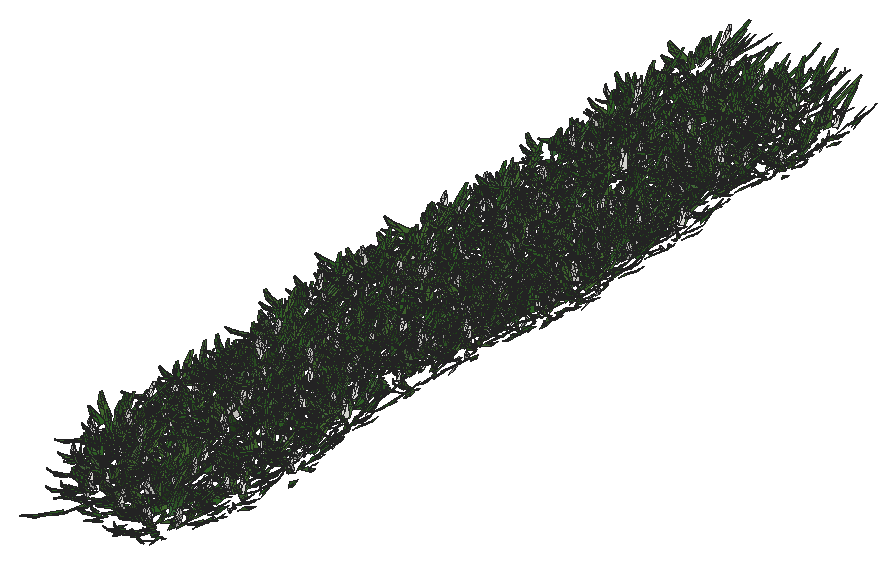
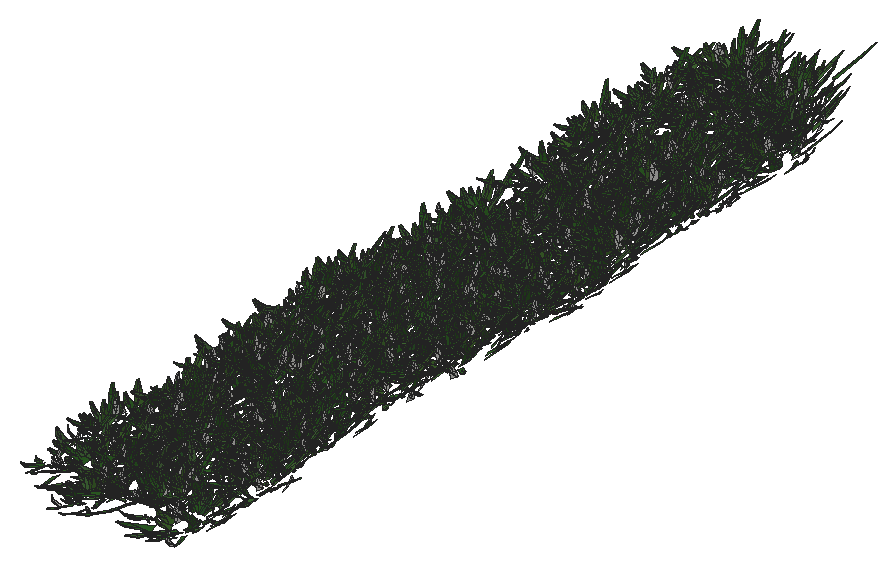
# SketchUp Ruby script. Lengths in inches.
U = 1.inch
M = Sketchup.active_model
def pt(a) = Geom::Point3d.new(a.map { |v| v * U })
def face(e, loops, mat)
  f = e.add_face(loops[0].map { |a| pt(a) })
  loops[1..].each { |l| e.add_face(l.map { |a| pt(a) }).erase! }
  f.material = f.back_material = mat if mat
  f
end
# faces: each face lists its corners as indices into pts; further lists are holes
def faces(e, pts, list, mat = nil) = list.each { |f| face(e, (f[0].is_a?(Array) ? f : [f]).map { |l| l.map { |i| pts[i] } }, mat) }
# xy, xz, yz: faces in a plane at the given z, y or x. An outline is a flat list of corners, or four numbers for a rectangle; further outlines are holes
def ring(l) = l.size == 4 ? [[l[0], l[1]], [l[2], l[1]], [l[2], l[3]], [l[0], l[3]]] : l.each_slice(2).to_a
def flat(e, list, mat, &to3) = list.each { |f| face(e, (f[0].is_a?(Array) ? f : [f]).map { |l| ring(l).map { |u, v| to3.(u, v) } }, mat) }
def xy(e, z, list, mat = nil) = flat(e, list, mat) { |x, y| [x, y, z] }
def xz(e, y, list, mat = nil) = flat(e, list, mat) { |x, z| [x, y, z] }
def yz(e, x, list, mat = nil) = flat(e, list, mat) { |y, z| [x, y, z] }
def lines(e, pts, list) = list.each { |a, b| e.add_line(pt(pts[a]), pt(pts[b])) }
# prism: a flat outline (further loops are holes) pulled along v
def prism(e, loops, v, mat = nil)
  f = face(e, loops, mat); d = Geom::Vector3d.new(v.map { |x| x * U })
  f.pushpull(f.normal.samedirection?(d) ? d.length : -d.length)
end
def box(e, o, s, mat = nil) = prism(e, [[o, [o[0] + s[0], o[1], o[2]], [o[0] + s[0], o[1] + s[1], o[2]], [o[0], o[1] + s[1], o[2]]]], [0, 0, s[2]], mat)
def at(x, y, z, deg = 0) = Geom::Transformation.translation(pt([x, y, z])) * Geom::Transformation.rotation(ORIGIN, Z_AXIS, deg.degrees)
def axes(o, x, y, z) = Geom::Transformation.new([*x, 0, *y, 0, *z, 0, *pt(o).to_a, 1])
def part(name) = M.definitions.add(name)
# library, detail: a bought-in or finely detailed component or shape, given as its bounding box
def library(name, o, s) = part(name).tap { |d| box(d.entities, o, s) }
def detail(e, o, s) = box(e.add_group.entities, o, s)
def put(e, d, t, mat = nil) = e.add_instance(d, t).tap { |i| i.material = mat if mat }
def group(e, t, mat = nil) = e.add_group.tap { |g| g.transformation = t; g.material = mat if mat }.entities
root = M.entities
M.materials.add("Material10").color = [48, 90, 38]
M.materials.add("Material11").color = [68, 110, 48]
M.materials.add("Material12").color = [48, 90, 48]
M.materials.add("Material13").color = [58, 110, 58]
M.materials.add("Material14").color = [58, 90, 38]
M.materials.add("Material15").color = [68, 100, 58]
M.materials.add("Material16").color = [48, 100, 38]
M.materials.add("Material9").color = [68, 110, 58]
c1 = part("grass00")
p = [[-0.6875,0.15,0],[-0.56,0.08,5.52],[-0.04,0.03,2.76],[0.48,-0.02,0],[0.35,-0.02,5.52],[-0.1,-0.14,5.52],
  [-0.12,0.65,8.37],[-0.42,0.65,8.37]]
faces(c1.entities,p,[[0,1,2,3],[3,2,4],[1,5,2],[5,4,2],[1,6,5],[4,5,6],[7,6,1]])
c2 = part("Group16\#1")
put(c2.entities,c1,axes([1.44,-0.61,-0.01],[0.05352,0.12609,0],[-0.10704,0.04543,0.07239],[0.06664,-0.02828,0.11628]),"Material12")
put(c2.entities,c1,axes([0.76,-0.15,-0.01],[0.04676,0.24062,0],[-0.23162,0.04501,0.06642],[0.0652,-0.01267,0.23595]),"Material9")
put(c2.entities,c1,axes([0.79,0.01,-0.01],[-0.00606,0.34651,0],[-0.34381,-0.00602,0.0432],[0.04319,0.00076,0.34386]))
put(c2.entities,c1,axes([1,0.23,-0.01],[-0.07192,0.31144,0],[-0.28722,-0.06632,0.1236],[0.12043,0.02781,0.29478]),"Material11")
put(c2.entities,c1,axes([1.66,0.77,-0.01],[-0.13828,0.29651,0],[-0.21551,-0.1005,0.22471],[0.20365,0.09498,0.23779]),"Material16")
put(c2.entities,c1,axes([0.6875,0.52,-0.01],[-0.18126,0.24051,0],[-0.22746,-0.17142,0.09788],[0.07817,0.05891,0.28481]),"Material11")
put(c2.entities,c1,axes([0.68,0.78,-0.01],[-0.215,0.18688,0],[-0.12385,-0.14248,0.21334],[0.13995,0.16101,0.18878]),"Material9")
put(c2.entities,c1,axes([0.56,1,-0.01],[-0.13756,0.07624,0],[-0.06159,-0.11112,0.0927],[0.04494,0.08108,0.12705]),"Material11")
put(c2.entities,c1,axes([0.2,0.64,-0.01],[-0.23729,0.07254,0],[-0.05711,-0.18681,0.153],[0.04473,0.14632,0.19535]),"Material16")
put(c2.entities,c1,axes([0.0625,0.72,-0.01],[-0.28874,0.02525,0],[-0.02179,-0.24916,0.14647],[0.01276,0.14591,0.25012]),"Material9")
put(c2.entities,c1,axes([-0.08,0.62,-0.01],[-0.34089,-0.04187,0],[0.03255,-0.26504,0.216],[-0.02633,0.21439,0.26703]),"Material16")
put(c2.entities,c1,axes([-0.34,0.98,-0.01],[-0.14314,-0.0493,0],[0.04397,-0.12769,0.06843],[-0.02228,0.0647,0.13505]),"Material16")
put(c2.entities,c1,axes([-0.87,1.45,-0.01],[-0.23488,-0.14114,0],[0.13761,-0.22901,0.06087],[-0.03135,0.05217,0.26717]))
put(c2.entities,c1,axes([-0.72,0.77,-0.01],[-0.14208,-0.13251,0],[0.07209,-0.0773,0.16301],[-0.11118,0.11922,0.1057]),"Material16")
put(c2.entities,c1,axes([-0.62,0.43,-0.01],[-0.14845,-0.21203,0],[0.18654,-0.13061,0.12304],[-0.10079,0.07057,0.22772]),"Material9")
put(c2.entities,c1,axes([-0.68,0.29,-0.01],[-0.13639,-0.32136,0],[0.31723,-0.13464,0.05579],[-0.05136,0.0218,0.34462]),"Material10")
put(c2.entities,c1,axes([-0.64,0.125,-0.01],[-0.0458,-0.23569,0],[0.22124,-0.043,0.08276],[-0.08124,0.01579,0.22538]),"Material13")
put(c2.entities,c1,axes([-1.6,-0.03,-0.01],[0.00576,-0.32897,0],[0.27526,0.00482,0.18018],[-0.18015,-0.00315,0.2753]),"Material11")
put(c2.entities,c1,axes([-1.36,-0.31,-0.01],[0.05718,-0.24765,0],[0.18172,0.04196,0.17267],[-0.16825,-0.03885,0.1865]),"Material16")
put(c2.entities,c1,axes([-1.54,-0.72,-0.01],[0.06537,-0.14017,0],[0.13555,0.06321,0.03939],[-0.0357,-0.01665,0.14956]))
put(c2.entities,c1,axes([-1.19,-0.9,-0.01],[0.09597,-0.12735,0],[0.11214,0.08451,0.07557],[-0.06035,-0.04548,0.14042]),"Material15")
put(c2.entities,c1,axes([-0.47,-0.54,-0.01],[0.11588,-0.10072,0],[0.0618,0.0711,0.12124],[-0.07953,-0.0915,0.0942]))
put(c2.entities,c1,axes([-0.47,-0.84,-0.01],[0.11927,-0.0661,0],[0.06603,0.11913,0.00646],[-0.00313,-0.00565,0.13621]),"Material11")
put(c2.entities,c1,axes([-0.38,-1.24,-0.01],[0.28037,-0.08571,0],[0.0618,0.20215,0.20315],[-0.05939,-0.19428,0.21139]),"Material15")
put(c2.entities,c1,axes([-0.06,-0.66,-0.01],[0.22719,-0.01987,0],[0.01247,0.14255,0.17758],[-0.01547,-0.17691,0.1431]),"Material14")
put(c2.entities,c1,axes([0.11,-0.89,-0.01],[0.14882,0.01828,0],[-0.01058,0.08611,0.12229],[0.01491,-0.12138,0.08676]),"Material12")
put(c2.entities,c1,axes([0.25,-0.72,-0.01],[0.20481,0.07053,0],[-0.06206,0.18022,0.10291],[0.03351,-0.0973,0.1906]),"Material12")
put(c2.entities,c1,axes([0.85,-1.42,-0.01],[0.16481,0.09904,0],[-0.09472,0.15762,0.05616],[0.02893,-0.04814,0.18389]),"Material11")
put(c2.entities,c1,axes([1.01,-1.09,-0.01],[0.21858,0.20385,0],[-0.17495,0.1876,0.15339],[0.10462,-0.11218,0.25652]),"Material16")
put(c2.entities,c1,axes([1.01,-0.71,-0.01],[0.08733,0.12473,0],[-0.06445,0.04512,0.13037],[0.1068,-0.07477,0.07867]),"Material12")
c3 = part("Group15\#1")
put(c3.entities,c2,at(0,0,0))
c4 = part("3darcstudiotree_grass00\#1")
put(c4.entities,c3,at(0,0,0))
put(root,c4,axes([846.08,365.22,12.99],[1.06369,-5.76804,0],[2.34649,2.26106,-0.03331],[0.13333,0.12847,1.51731]))
put(root,c4,axes([846.18,479.74,12.99],[0.45259,5.87694,0],[-3.26833,1.31518,-0.06022],[-0.23227,0.09347,1.78296]))
put(root,c4,axes([846.2,370.94,12.99],[1.45402,4.55379,0],[-2.35041,3.92143,-0.05552],[-0.15671,0.26146,1.39481]))
put(root,c4,axes([847.63,497.58,12.99],[-1.00824,-6.55152,0],[2.51742,-2.02434,-0.03242],[0.11179,-0.0899,1.33794]))
put(root,c4,axes([848.5,380.8125,12.99],[-3.32323,0.92593,0],[-0.32804,-6.15195,-0.03065],[-0.01972,-0.36975,1.97713]))
put(root,c4,axes([848.83,465.13,12.99],[-2.33029,-1.96474,0],[1.16034,-7.19112,-0.02933],[0.03799,-0.23541,1.72129]))
put(root,c4,axes([847.89,502.63,12.99],[3.21155,0.85953,0],[-0.39145,7.64247,-0.02723],[-0.01102,0.21518,1.60719]))
put(root,c4,axes([848.18,289.78,12.99],[2.86445,-0.82084,0],[0.41094,7.49322,-0.03701],[0.02027,0.36959,1.99511]))
put(root,c4,axes([848,405.99,12.99],[2.95868,3.40563,0],[-1.44175,6.54478,-0.03278],[-0.06316,0.28671,1.8841]))
put(root,c4,axes([848.98,375.9,12.99],[1.21855,-5.78751,0],[3.1286,3.44196,-0.06017],[0.19802,0.21785,1.73941]))
put(root,c4,axes([848.31,448.79,12.99],[2.69698,1.04179,0],[-0.45125,6.10404,-0.04218],[-0.0351,0.4748,1.85529]))
put(root,c4,axes([849.4,316.99,12.99],[-0.81503,-5.65935,0],[3.10311,-2.33512,-0.05688],[0.2199,-0.16548,1.82396]))
put(root,c4,axes([848.26,357.72,12.99],[3.10556,1.6743,0],[-0.67424,6.53475,-0.02883],[-0.03024,0.29312,1.84132]))
put(root,c4,axes([848.99,310.21,12.99],[2.13184,-3.94964,0],[2.03475,5.73869,-0.02341],[0.0529,0.14921,1.59067]))
put(root,c4,axes([849.87,327.62,12.99],[-2.25962,-3.55393,0],[1.58703,-5.27249,-0.02104],[0.05386,-0.17895,1.73448]))
put(root,c4,axes([849.875,457.09,12.99],[-1.95242,-3.89116,0],[1.88937,-4.95355,-0.03875],[0.11017,-0.28885,1.70607]))
put(root,c4,axes([849.33,346.31,12.99],[1.84633,-3.73447,0],[2.12858,5.4989,-0.04815],[0.14229,0.36759,1.9649]))
put(root,c4,axes([849.15,475.27,12.99],[2.63938,2.75355,0],[-1.03955,5.20668,-0.03533],[-0.07966,0.39899,1.86502]))
put(root,c4,axes([849.78,394.45,12.99],[2.77698,1.25039,0],[-0.63996,7.42652,-0.03192],[-0.01976,0.22931,1.45488]))
put(root,c4,axes([850.04,428.51,12.99],[-0.33187,6.17881,0],[-2.97957,-0.83623,-0.03564],[-0.14689,-0.04123,1.71014]))
put(root,c4,axes([849.88,423.01,12.99],[1.88972,4.62995,0],[-2.56011,5.45989,-0.03325],[-0.08097,0.17268,1.59934]))
put(root,c4,axes([851.5,405.58,12.99],[0.21539,-7.71794,0],[2.95559,0.431,-0.05413],[0.18491,0.02696,1.39055]))
put(root,c4,axes([851.65,343.35,12.99],[0.44599,-7.88278,0],[3.43149,1.01446,-0.05291],[0.14746,0.0436,1.33374]))
put(root,c4,axes([851.93,393.51,12.99],[1.99767,-5.75199,0],[2.71363,4.92449,-0.06314],[0.13539,0.2457,1.30132]))
put(root,c4,axes([852,321.69,12.99],[0.51895,6.13984,0],[-2.64873,1.16979,-0.03785],[-0.14312,0.06321,1.42505]))
put(root,c4,axes([853.47,336.67,12.99],[-2.97565,-3.89676,0],[1.54592,-6.16836,-0.04075],[0.07384,-0.29465,1.55523]))
put(root,c4,axes([853.5,456.88,12.99],[-0.62688,-5.64888,0],[2.8559,-1.65605,-0.05601],[0.24214,-0.14041,1.80254]))
put(root,c4,axes([853.51,386.74,12.99],[1.87221,-4.7946,0],[2.54876,5.20039,-0.02458],[0.06994,0.14271,1.78746]))
put(root,c4,axes([854.24,441.14,12.99],[-2.80442,-2.07275,0],[1.02319,-7.23363,-0.04655],[0.0496,-0.35067,1.58019]))
put(root,c4,axes([853.31,288.82,12.99],[2.65285,-1.87873,0],[0.74671,5.50944,-0.04073],[0.05006,0.36938,1.43775]))
put(root,c4,axes([853.33,281.66,12.99],[1.13363,5.60093,0],[-3.05552,3.23148,-0.03574],[-0.13437,0.1421,1.91331]))
put(root,c4,axes([853.67,468.9,12.99],[3.14674,3.47141,0],[-1.27001,6.01543,-0.05424],[-0.08028,0.38023,1.36476]))
put(root,c4,axes([854.51,371.89,12.99],[0.93873,-6.42371,0],[2.31185,1.76531,-0.03453],[0.17252,0.13174,1.76116]))
put(root,c4,axes([854.56,274.28,12.99],[0.65379,5.49988,0],[-2.52465,1.56816,-0.02204],[-0.11086,0.06886,1.87051]))
put(root,c4,axes([855.72,335.64,12.99],[-3.16702,-0.15371,0],[0.065,-6.99788,-0.04949],[0.00478,-0.51432,1.9102]))
put(root,c4,axes([856.45,461.74,12.99],[-1.32807,-5.2436,0],[2.60307,-3.44493,-0.02105],[0.08579,-0.11354,1.94345]))
put(root,c4,axes([856.77,439.38,12.99],[-1.64718,-5.90379,0],[2.56899,-3.74523,-0.04256],[0.13378,-0.19503,1.55835]))
put(root,c4,axes([855.86,488.52,12.99],[2.4677,-0.18322,0],[0.11122,7.82696,-0.05593],[0.0062,0.43627,1.60461]))
put(root,c4,axes([857.21,498.3,12.99],[-0.46545,-5.51402,0],[3.35853,-1.48134,-0.02161],[0.08848,-0.03903,1.95654]))
put(root,c4,axes([856.1,422.64,12.99],[0.68004,5.56927,0],[-2.40844,1.53666,-0.02635],[-0.10703,0.06829,1.4463]))
put(root,c4,axes([856.125,412.66,12.99],[2.75541,4.09981,0],[-1.44402,5.07109,-0.02904],[-0.07736,0.27168,1.7729]))
put(root,c4,axes([856.4,348.9375,12.99],[2.26086,2.51617,0],[-1.50969,7.08808,-0.05845],[-0.08327,0.39093,1.53958]))
put(root,c4,axes([857.63,307.67,12.99],[-3.30927,2.34914,0],[-0.81792,-6.02062,-0.03919],[-0.05215,-0.38386,1.69748]))
put(root,c4,axes([856.8,384.55,12.99],[2.97213,-0.50695,0],[0.20315,6.22325,-0.02534],[0.00797,0.24406,1.58232]))
put(root,c4,axes([857.21,283.69,12.99],[2.64295,-1.66108,0],[0.70112,5.82902,-0.03828],[0.04397,0.36554,1.57185]))
put(root,c4,axes([857.09,396.49,12.99],[2.73919,1.69577,0],[-0.71084,5.99975,-0.0432],[-0.04593,0.38771,1.51727]))
put(root,c4,axes([857.64,291.9375,12.99],[-1.59312,5.61237,0],[-2.64617,-3.92486,-0.05659],[-0.15346,-0.22762,1.39892]))
put(root,c4,axes([858.4375,374.95,12.99],[2.07615,-3.40292,0],[1.74164,5.55226,-0.04704],[0.11406,0.36363,1.70604]))
put(root,c4,axes([858.44,354.125,12.99],[3.18751,0.943,0],[-0.44534,7.86574,-0.04718],[-0.01874,0.3309,1.4726]))
put(root,c4,axes([858.63,299.875,12.99],[0.62532,7.4975,0],[-2.55479,1.11339,-0.03349],[-0.14821,0.06459,1.60736]))
put(root,c4,axes([858.61,328.54,12.99],[2.78691,3.36476,0],[-1.29729,5.61451,-0.05015],[-0.11211,0.48519,1.82381]))
put(root,c4,axes([859.75,387.16,12.99],[2.35938,-4.85445,0],[1.80036,4.57218,-0.02235],[0.07834,0.19896,1.93391]))
put(root,c4,axes([860.79,269.33,12.99],[1.03895,-7.06461,0],[3.15067,2.42111,-0.02131],[0.07526,0.05783,1.69918]))
put(root,c4,axes([860.32,329.62,12.99],[1.78329,-6.04262,0],[2.25042,3.47028,-0.04469],[0.18181,0.28036,1.8275]))
put(root,c4,axes([861.14,403.99,12.99],[-2.1541,-4.78139,0],[1.96653,-4.62931,-0.03796],[0.10802,-0.25428,1.58175]))
put(root,c4,axes([859.98,466.62,12.99],[-0.03905,5.59302,0],[-3.37157,-0.123,-0.04794],[-0.17064,-0.00623,1.64652]))
put(root,c4,axes([860.78,417.76,12.99],[1.18779,-6.50536,0],[2.63647,2.51534,-0.05171],[0.20007,0.19088,1.64301]))
put(root,c4,axes([860.42,484.72,12.99],[0.34647,5.87607,0],[-3.16065,0.97379,-0.05207],[-0.21092,0.06498,1.7882]))
put(root,c4,axes([861.61,306.74,12.99],[-2.22021,-5.6511,0],[2.49209,-5.11599,-0.05274],[0.16966,-0.34829,1.98669]))
put(root,c4,axes([860.97,456.35,12.99],[3,1.63244,0],[-0.75172,7.21848,-0.06215],[-0.05278,0.50679,1.63292]))
put(root,c4,axes([862.3125,429.31,12.99],[-2.4368,-3.09441,0],[1.60655,-6.61061,-0.02959],[0.05226,-0.21506,1.65043]))
put(root,c4,axes([861.14,450.09,12.99],[1.09008,5.94814,0],[-2.83436,2.71417,-0.03717],[-0.13159,0.12601,1.61797]))
put(root,c4,axes([861.15,365.25,12.99],[2.15587,4.20517,0],[-1.86376,4.99268,-0.03219],[-0.10025,0.26855,1.88986]))
put(root,c4,axes([862.625,440.88,12.99],[-3.26232,-2.86014,0],[1.20503,-7.18193,-0.02874],[0.02985,-0.17791,1.33872]))
put(root,c4,axes([862.22,338.99,12.99],[3.03096,-2.26489,0],[0.92784,6.488,-0.04269],[0.06267,0.43825,1.93529]))
put(root,c4,axes([862.67,317.89,12.99],[2.03931,-4.55463,0],[2.25979,5.28691,-0.03867],[0.1061,0.24824,1.7417]))
put(root,c4,axes([864.13,401.76,12.99],[-2.91157,-4.36753,0],[1.37492,-4.78932,-0.04657],[0.13679,-0.47648,1.84036]))
put(root,c4,axes([863.91,270.64,12.99],[0.97376,-6.54554,0],[2.91638,2.26702,-0.01889],[0.08323,0.0647,1.96679]))
put(root,c4,axes([863.84,430.42,12.99],[1.88791,-4.76604,0],[2.09608,4.33845,-0.04299],[0.13117,0.27149,1.59659]))
put(root,c4,axes([864.51,264.94,12.99],[-2.24252,-6.03591,0],[2.28388,-4.43375,-0.05304],[0.19219,-0.37311,1.95407]))
put(root,c4,axes([863.99,449.02,12.99],[-1.55822,6.01772,0],[-2.59774,-3.51477,-0.03668],[-0.15095,-0.20424,1.98009]))
put(root,c4,axes([864.28,343.09,12.99],[-2.29812,5.55657,0],[-1.95842,-4.23231,-0.02847],[-0.07859,-0.16983,1.40417]))
put(root,c4,axes([865.0625,385.5625,12.99],[-3.35624,0.65398,0],[-0.22542,-6.04474,-0.04632],[-0.02051,-0.54987,1.89764]))
put(root,c4,axes([865.07,419.13,12.99],[-0.90881,5.87798,0],[-2.31035,-1.86649,-0.03966],[-0.15425,-0.12462,1.38647]))
put(root,c4,axes([865.43,367.76,12.99],[-2.58772,5.27673,0],[-1.86753,-4.78548,-0.04505],[-0.10853,-0.2781,1.39266]))
put(root,c4,axes([866.125,408.51,12.99],[-1.00456,-5.95255,0],[2.82963,-2.49521,-0.03571],[0.15413,-0.13592,1.92492]))
put(root,c4,axes([865.09,496.71,12.99],[1.44814,6.075,0],[-2.47408,3.08166,-0.025],[-0.11319,0.14099,1.99255]))
put(root,c4,axes([866.3125,374.3,12.99],[-3.03706,0.21927,0],[-0.09301,-6.73134,-0.03959],[-0.00511,-0.36973,1.65212]))
put(root,c4,axes([865.2,333.54,12.99],[2.0574,6.068,0],[-2.66536,4.72208,-0.03267],[-0.1083,0.19187,1.93988]))
put(root,c4,axes([865.32,480.65,12.99],[1.0519,6.52766,0],[-3.10051,2.61067,-0.04046],[-0.13074,0.11008,1.56076]))
put(root,c4,axes([865.4,315.18,12.99],[0.01985,5.9818,0],[-3.45212,0.05986,-0.03677],[-0.10753,0.00186,1.38481]))
put(root,c4,axes([866.68,280.02,12.99],[-2.88358,-0.6118,0],[0.31664,-7.79826,-0.06502],[0.01826,-0.44966,1.42798]))
put(root,c4,axes([866.74,308.83,12.99],[1.01643,-7.0272,0],[3.11902,2.35731,-0.04027],[0.1453,0.10982,1.71232]))
put(root,c4,axes([868.36,363.89,12.99],[-0.70141,-5.97923,0],[3.35556,-2.05683,-0.04199],[0.15153,-0.09288,1.7807]))
put(root,c4,axes([868.625,391.23,12.99],[-1.89539,-4.49691,0],[2.16024,-4.75765,-0.03217],[0.08926,-0.19659,1.58546]))
put(root,c4,axes([868.4,308.07,12.99],[-3.1313,1.31472,0],[-0.62999,-7.8402,-0.05609],[-0.04113,-0.51187,1.94158]))
put(root,c4,axes([868.59,349.82,12.99],[-2.83779,-3.28018,0],[1.1007,-4.97574,-0.0255],[0.06682,-0.30206,1.94297]))
put(root,c4,axes([868.34,470.72,12.99],[-2.63853,4.19895,0],[-1.87852,-6.16795,-0.02528],[-0.05662,-0.18591,1.76765]))
put(root,c4,axes([868.16,292.33,12.99],[0.10307,6.4841,0],[-2.60811,0.21663,-0.04285],[-0.21858,0.01816,1.82733]))
put(root,c4,axes([868.29,460.95,12.99],[2.50531,-1.67127,0],[0.93841,7.35041,-0.04654],[0.03812,0.29858,1.34343]))
put(root,c4,axes([868.1,495.49,12.99],[2.68458,2.75681,0],[-1.10476,5.62136,-0.04301],[-0.08005,0.40733,1.6797]))
put(root,c4,axes([868.52,353.45,12.99],[2.60889,-2.1734,0],[1.10499,6.93076,-0.06136],[0.08576,0.53791,1.80687]))
put(root,c4,axes([869.98,284.06,12.99],[-3.1777,2.21789,0],[-0.99385,-7.44046,-0.03433],[-0.02906,-0.21757,1.35329]))
put(root,c4,axes([869.83,408.75,12.99],[-2.2266,5.00695,0],[-1.83096,-4.25454,-0.0233],[-0.08368,-0.19444,1.83382]))
put(root,c4,axes([869.87,327.39,12.99],[-0.4769,5.50254,0],[-3.02986,-1.37211,-0.03573],[-0.13861,-0.06277,1.67549]))
put(root,c4,axes([870.34,372.19,12.99],[-0.6659,7.19493,0],[-3.288,-1.59009,-0.05558],[-0.1877,-0.09077,1.59125]))
put(root,c4,axes([870.86,475.71,12.99],[1.24347,-6.30598,0],[2.24288,2.31096,-0.02223],[0.09784,0.10081,1.62899]))
put(root,c4,axes([872.16,348.43,12.99],[-1.18537,-5.54659,0],[2.44574,-2.73113,-0.0349],[0.1548,-0.17286,1.84302]))
put(root,c4,axes([872.59,405.5,12.99],[-2.8541,-0.0395,0],[0.02062,-7.78505,-0.0591],[0.00117,-0.44044,1.52309]))
put(root,c4,axes([872.74,387.25,12.99],[-3.17891,-0.60485,0],[0.24844,-6.82268,-0.036],[0.01418,-0.38953,1.9513]))
put(root,c4,axes([872.64,506.55,12.99],[0.98174,-5.21568,0],[2.70185,2.65738,-0.02985],[0.10494,0.10321,1.54439]))
put(root,c4,axes([872.42,436.46,12.99],[0.61942,-5.96717,0],[2.37092,1.286,-0.04624],[0.26261,0.14244,1.95114]))
put(root,c4,axes([872.41,478.23,12.99],[-1.50219,6.01734,0],[-2.18613,-2.85168,-0.04437],[-0.16348,-0.21326,1.46464]))
put(root,c4,axes([873.08,264.28,12.99],[0.90473,-6.6234,0],[3.21141,2.29213,-0.04262],[0.16012,0.11428,1.81655]))
put(root,c4,axes([873.125,318.22,12.99],[-1.81586,6.81794,0],[-2.31926,-3.22763,-0.03488],[-0.10964,-0.15258,1.37068]))
put(root,c4,axes([872.79,339.07,12.99],[2.50071,-0.75735,0],[0.34878,6.01755,-0.04905],[0.02621,0.45221,1.48186]))
put(root,c4,axes([873.25,283.78,12.99],[2.37117,-2.04607,0],[0.95251,5.76786,-0.04981],[0.08018,0.48553,1.68613]))
put(root,c4,axes([874.18,395.51,12.99],[-1.52422,-6.19086,0],[2.53637,-3.26297,-0.05229],[0.18805,-0.24192,1.64764]))
put(root,c4,axes([874.25,327.95,12.99],[0.30354,-5.67688,0],[3.18511,0.8899,-0.02785],[0.09403,0.02627,1.49696]))
put(root,c4,axes([873.58,356.19,12.99],[-1.62139,7.1048,0],[-2.97912,-3.55246,-0.04188],[-0.152,-0.18125,1.88687]))
put(root,c4,axes([873.13,450.1,12.99],[2.13282,3.97865,0],[-1.89051,5.29544,-0.03119],[-0.09156,0.25647,1.90467]))
put(root,c4,axes([873.97,496.93,12.99],[-1.35304,6.81193,0],[-2.25958,-2.34517,-0.0444],[-0.19334,-0.20067,1.62807]))
put(root,c4,axes([874.22,418.82,12.99],[-1.67634,5.8436,0],[-2.79431,-4.18852,-0.05216],[-0.12461,-0.18678,1.30947]))
put(root,c4,axes([874.22,427.97,12.99],[-1.36273,6.90676,0],[-3.15633,-3.25402,-0.03185],[-0.11129,-0.11473,1.82087]))
put(root,c4,axes([874.28,309.18,12.99],[1.53536,4.3387,0],[-1.94807,3.60213,-0.02717],[-0.11192,0.20694,1.82093]))
put(root,c4,axes([874.36,271.34,12.99],[2.55774,1.63282,0],[-0.65651,5.37358,-0.03829],[-0.04318,0.35346,1.40372]))
put(root,c4,axes([874.74,469.97,12.99],[2.93849,-1.27374,0],[0.64821,7.81379,-0.05959],[0.03631,0.43776,1.56123]))
put(root,c4,axes([874.83,484.42,12.99],[0.60231,7.5978,0],[-3.28321,1.35999,-0.02342],[-0.08595,0.0356,1.70718]))
put(root,c4,axes([876.38,269.85,12.99],[-2.66911,-1.68953,0],[0.88763,-7.32722,-0.02644],[0.02949,-0.24342,1.9068]))
put(root,c4,axes([876.91,440.8,12.99],[-2.87219,-3.40969,0],[1.49679,-6.58817,-0.03725],[0.05993,-0.26378,1.55507]))
put(root,c4,axes([876.32,495.27,12.99],[-2.0005,6.23176,0],[-2.68773,-4.50835,-0.06171],[-0.18748,-0.31448,1.72322]))
put(root,c4,axes([876.13,465.47,12.99],[1.26204,4.81756,0],[-2.1346,2.92191,-0.04808],[-0.22521,0.30828,1.86326]))
put(root,c4,axes([876.11,391.07,12.99],[3.24405,-0.90953,0],[0.31828,5.93172,-0.03723],[0.01655,0.30849,1.30959]))
put(root,c4,axes([877.49,404.12,12.99],[-1.60999,-5.29002,0],[2.62708,-4.17777,-0.03629],[0.0981,-0.156,1.44541]))
put(root,c4,axes([877.5625,383.13,12.99],[-1.72268,-4.15908,0],[2.53682,-5.49039,-0.06171],[0.15262,-0.3303,1.63202]))
put(root,c4,axes([877.53,431.28,12.99],[-2.01727,3.38084,0],[-1.50139,-4.68098,-0.03589],[-0.1176,-0.36666,1.93035]))
put(root,c4,axes([877.49,414.09,12.99],[-1.11528,6.38022,0],[-2.67266,-2.44117,-0.0529],[-0.19703,-0.17997,1.58349]))
put(root,c4,axes([877.12,334.69,12.99],[1.02935,6.07343,0],[-2.35562,2.08612,-0.02409],[-0.10419,0.09227,1.60735]))
put(root,c4,axes([877.03,281.8125,12.99],[3.38432,1.80751,0],[-0.5848,5.72145,-0.04207],[-0.0361,0.3532,1.32997]))
put(root,c4,axes([877.95,316.04,12.99],[-2.06128,5.86676,0],[-2.13442,-3.91853,-0.04358],[-0.15088,-0.277,1.66757]))
put(root,c4,axes([877.4375,373.4,12.99],[2.65432,2.40211,0],[-1.03276,5.96302,-0.03237],[-0.05058,0.29202,1.63378]))
put(root,c4,axes([878.125,362.29,12.99],[2.50682,-4.9272,0],[1.58586,4.21591,-0.0226],[0.07323,0.19467,1.65792]))
put(root,c4,axes([878.96,461.24,12.99],[-3.11733,-0.19996,0],[0.07131,-5.80879,-0.03959],[0.00625,-0.50912,1.96257]))
put(root,c4,axes([877.83,356.16,12.99],[3.03118,3.59068,0],[-1.5694,6.92267,-0.0509],[-0.08069,0.3559,1.61215]))
put(root,c4,axes([879.01,327.69,12.99],[2.27046,-2.45056,0],[1.18742,5.74855,-0.03456],[0.06449,0.31223,1.66747]))
put(root,c4,axes([879.08,483.8,12.99],[-0.56033,5.43449,0],[-2.42934,-1.3088,-0.04738],[-0.19451,-0.10479,1.4441]))
put(root,c4,axes([880.56,421.96,12.99],[-2.61664,-2.33759,0],[0.99827,-5.83888,-0.02269],[0.03607,-0.21098,1.64292]))
put(root,c4,axes([880.28,263.08,12.99],[1.60465,-5.59865,0],[2.61478,3.91595,-0.04807],[0.15921,0.23843,1.69791]))
put(root,c4,axes([880.4,365.48,12.99],[1.86259,-5.03556,0],[2.26194,4.37174,-0.03628],[0.10162,0.19641,1.49031]))
put(root,c4,axes([880.99,456.66,12.99],[-1.25841,-6.18676,0],[2.25736,-2.3992,-0.04244],[0.21463,-0.22811,1.90455]))
put(root,c4,axes([881.86,372.23,12.99],[-1.4028,-6.63349,0],[2.73636,-3.02366,-0.04214],[0.14191,-0.15681,1.55921]))
put(root,c4,axes([881.32,465.27,12.99],[-2.21576,3.96026,0],[-1.7021,-4.9761,-0.02144],[-0.06774,-0.19804,1.94421]))
put(root,c4,axes([880.89,401.66,12.99],[-0.46879,6.13734,0],[-2.74621,-1.09606,-0.03794],[-0.13938,-0.05563,1.42617]))
put(root,c4,axes([881.3,297.27,12.99],[-1.39114,5.97998,0],[-2.29712,-2.79228,-0.04799],[-0.23659,-0.28759,1.99284]))
put(root,c4,axes([881.9,494.4,12.99],[0.14936,-7.38431,0],[3.15877,0.33386,-0.04434],[0.15811,0.01671,1.54852]))
put(root,c4,axes([881.89,431.37,12.99],[-1.68881,6.92938,0],[-2.83305,-3.60784,-0.0557],[-0.16956,-0.21593,1.55009]))
put(root,c4,axes([882.83,447.51,12.99],[-2.37222,-5.8724,0],[2.55146,-5.3856,-0.04946],[0.11321,-0.23896,1.48426]))
put(root,c4,axes([882.69,390.27,12.99],[-2.96814,-1.04488,0],[0.40182,-5.96422,-0.03709],[0.0263,-0.39033,1.68681]))
put(root,c4,axes([882.44,382.91,12.99],[-2.3067,2.43505,0],[-1.34707,-6.66775,-0.05064],[-0.07084,-0.35063,1.47033]))
put(root,c4,axes([882.92,436.65,12.99],[1.45497,-4.57491,0],[2.28679,3.80017,-0.02782],[0.10975,0.18238,1.89124]))
put(root,c4,axes([882.53,358.07,12.99],[1.76342,4.06356,0],[-2.21638,5.02573,-0.03885],[-0.10236,0.23211,1.58937]))
put(root,c4,axes([882.93,414.71,12.99],[2.2991,1.96197,0],[-1.09932,6.73127,-0.03179],[-0.04562,0.27936,1.76952]))
put(root,c4,axes([884.34,394.66,12.99],[-1.18442,-5.88193,0],[2.43707,-2.56425,-0.04546],[0.20078,-0.21126,1.78943]))
put(root,c4,axes([884.88,309.3125,12.99],[-2.69027,-2.5136,0],[0.9649,-5.39619,-0.04864],[0.07532,-0.42124,1.4319]))
put(root,c4,axes([884.98,436.55,12.99],[-1.2711,-5.87901,0],[3.04745,-3.44284,-0.04891],[0.17708,-0.20005,1.88309]))
put(root,c4,axes([884.84,299.1875,12.99],[-0.398,-6.92613,0],[2.57524,-0.77325,-0.04534],[0.20481,-0.0615,1.62314]))
put(root,c4,axes([885.41,380.5,12.99],[-0.92749,-6.3858,0],[2.74177,-2.0808,-0.03393],[0.10736,-0.08147,1.3212]))
put(root,c4,axes([884.6,263.125,12.99],[3.00894,-2.03191,0],[0.93466,7.23212,-0.05518],[0.06124,0.47388,1.77288]))
put(root,c4,axes([885.17,367.37,12.99],[-1.76112,4.57204,0],[-2.37853,-4.78733,-0.02335],[-0.0674,-0.13566,1.67208]))
put(root,c4,axes([885.49,457.58,12.99],[-2.54467,5.14028,0],[-2.10174,-5.43661,-0.04086],[-0.09075,-0.23474,1.46035]))
put(root,c4,axes([885.67,372,12.99],[1.85254,-5.66615,0],[2.17332,3.71286,-0.03861],[0.14629,0.24992,1.76068]))
put(root,c4,axes([886.23,286.94,12.99],[0.61763,-7.14229,0],[3.29961,1.49093,-0.04547],[0.16686,0.07539,1.72572]))
put(root,c4,axes([885.44,326.6,12.99],[2.60761,2.35938,0],[-0.9387,5.42096,-0.04887],[-0.09514,0.5494,1.85053]))
put(root,c4,axes([885.86,427.28,12.99],[0.94943,6.35721,0],[-2.57871,2.01236,-0.04031],[-0.1809,0.14117,1.77227]))
put(root,c4,axes([886.61,470.19,12.99],[-2.65013,2.01595,0],[-1.04623,-7.18648,-0.02244],[-0.0254,-0.17449,1.62972]))
put(root,c4,axes([886.86,349.46,12.99],[0.19702,-7.42843,0],[2.98539,0.41373,-0.02606],[0.10666,0.01478,1.68211]))
put(root,c4,axes([886.66,320.42,12.99],[-1.79207,5.80307,0],[-2.3887,-3.85447,-0.04566],[-0.15348,-0.24766,1.65042]))
put(root,c4,axes([887.22,422.87,12.99],[2.82086,-1.26593,0],[0.6014,7.00235,-0.02697],[0.01941,0.22601,1.59996]))
put(root,c4,axes([888.78,493.03,12.99],[-0.90122,7.47245,0],[-2.56603,-1.61709,-0.03305],[-0.11789,-0.0743,1.35106]))
put(root,c4,axes([889.2,413.43,12.99],[-1.50151,6.30487,0],[-2.86193,-3.56136,-0.05406],[-0.16351,-0.20347,1.53936]))
put(root,c4,axes([889.77,404.08,12.99],[-2.51057,2.58377,0],[-1.34342,-6.8208,-0.05685],[-0.09795,-0.49729,1.88376]))
put(root,c4,axes([889.28,278.0625,12.99],[-0.59528,6.16644,0],[-3.08896,-1.55812,-0.05256],[-0.15476,-0.07806,1.30827]))
put(root,c4,axes([889.88,479.93,12.99],[1.26802,-4.95481,0],[2.2898,3.06198,-0.02347],[0.10746,0.1437,1.9305]))
put(root,c4,axes([890.38,395.3,12.99],[-0.41112,-5.93893,0],[3.42722,-1.23966,-0.05346],[0.16372,-0.05922,1.47567]))
put(root,c4,axes([889.91,302.97,12.99],[1.70976,-6.14589,0],[2.21726,3.22309,-0.04064],[0.13956,0.20287,1.46692]))
put(root,c4,axes([889.46,386.59,12.99],[1.6634,5.16123,0],[-2.41338,4.06419,-0.0323],[-0.09461,0.15932,1.496]))
put(root,c4,axes([889.93,437.26,12.99],[-1.0347,5.85385,0],[-2.62739,-2.42663,-0.02451],[-0.09705,-0.08964,1.66036]))
